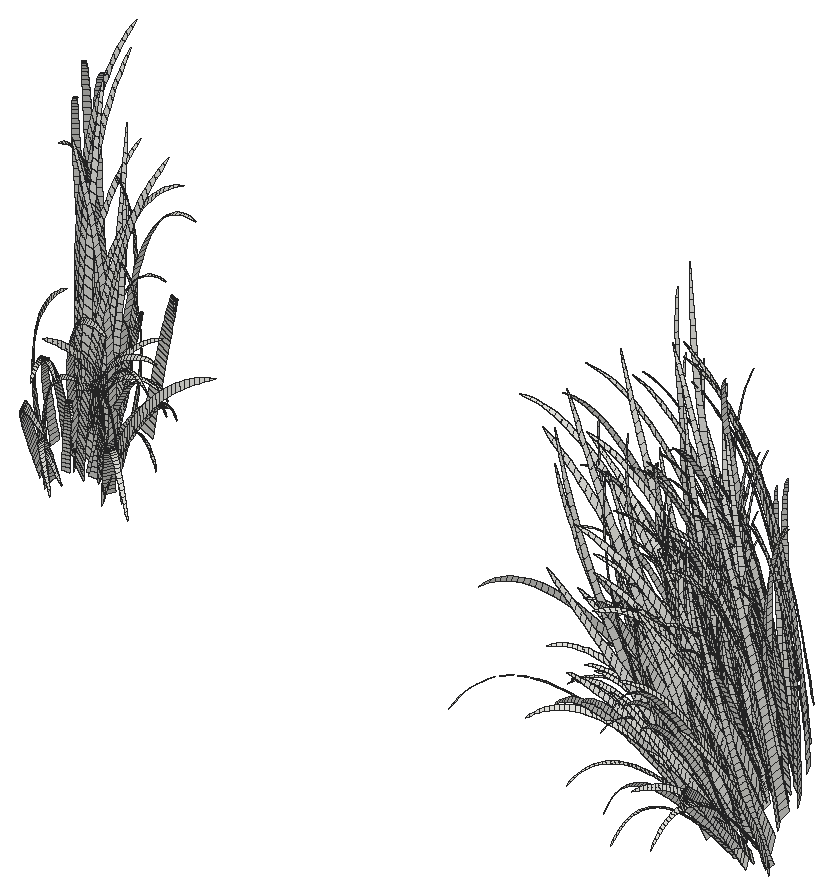
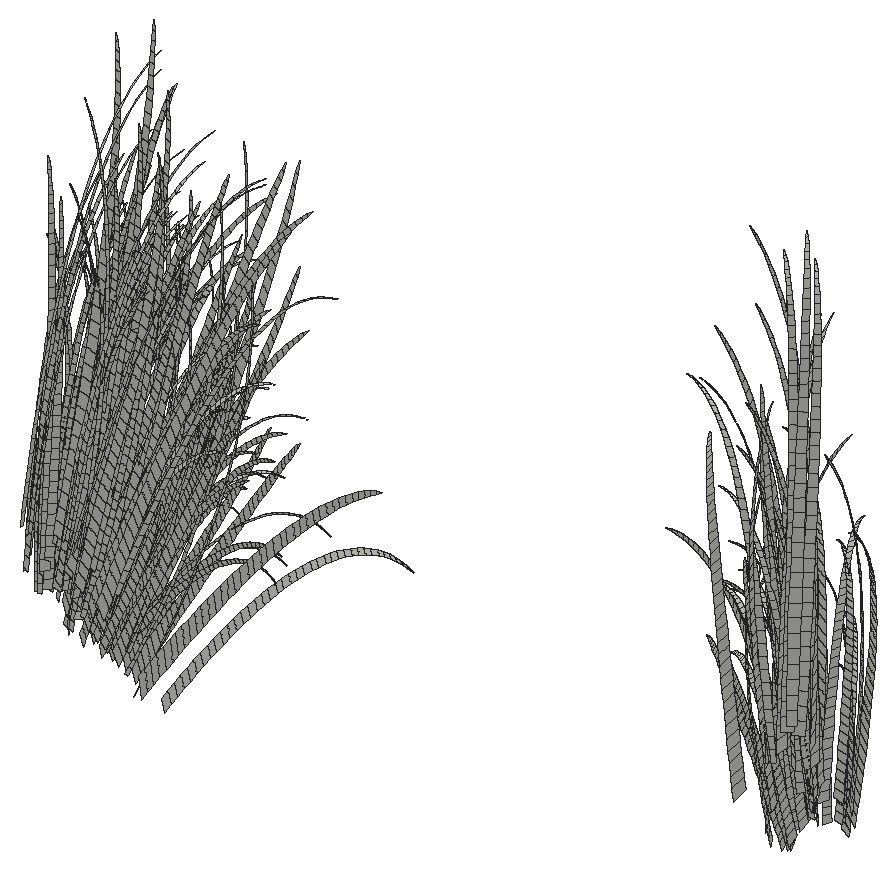
# SketchUp Ruby script. Lengths in inches.
U = 1.inch
M = Sketchup.active_model
def pt(a) = Geom::Point3d.new(a.map { |v| v * U })
def face(e, loops, mat)
  f = e.add_face(loops[0].map { |a| pt(a) })
  loops[1..].each { |l| e.add_face(l.map { |a| pt(a) }).erase! }
  f.material = f.back_material = mat if mat
  f
end
# faces: each face lists its corners as indices into pts; further lists are holes
def faces(e, pts, list, mat = nil) = list.each { |f| face(e, (f[0].is_a?(Array) ? f : [f]).map { |l| l.map { |i| pts[i] } }, mat) }
# xy, xz, yz: faces in a plane at the given z, y or x. An outline is a flat list of corners, or four numbers for a rectangle; further outlines are holes
def ring(l) = l.size == 4 ? [[l[0], l[1]], [l[2], l[1]], [l[2], l[3]], [l[0], l[3]]] : l.each_slice(2).to_a
def flat(e, list, mat, &to3) = list.each { |f| face(e, (f[0].is_a?(Array) ? f : [f]).map { |l| ring(l).map { |u, v| to3.(u, v) } }, mat) }
def xy(e, z, list, mat = nil) = flat(e, list, mat) { |x, y| [x, y, z] }
def xz(e, y, list, mat = nil) = flat(e, list, mat) { |x, z| [x, y, z] }
def yz(e, x, list, mat = nil) = flat(e, list, mat) { |y, z| [x, y, z] }
def lines(e, pts, list) = list.each { |a, b| e.add_line(pt(pts[a]), pt(pts[b])) }
# prism: a flat outline (further loops are holes) pulled along v
def prism(e, loops, v, mat = nil)
  f = face(e, loops, mat); d = Geom::Vector3d.new(v.map { |x| x * U })
  f.pushpull(f.normal.samedirection?(d) ? d.length : -d.length)
end
def box(e, o, s, mat = nil) = prism(e, [[o, [o[0] + s[0], o[1], o[2]], [o[0] + s[0], o[1] + s[1], o[2]], [o[0], o[1] + s[1], o[2]]]], [0, 0, s[2]], mat)
def at(x, y, z, deg = 0) = Geom::Transformation.translation(pt([x, y, z])) * Geom::Transformation.rotation(ORIGIN, Z_AXIS, deg.degrees)
def axes(o, x, y, z) = Geom::Transformation.new([*x, 0, *y, 0, *z, 0, *pt(o).to_a, 1])
def part(name) = M.definitions.add(name)
# library, detail: a bought-in or finely detailed component or shape, given as its bounding box
def library(name, o, s) = part(name).tap { |d| box(d.entities, o, s) }
def detail(e, o, s) = box(e.add_group.entities, o, s)
def put(e, d, t, mat = nil) = e.add_instance(d, t).tap { |i| i.material = mat if mat }
def group(e, t, mat = nil) = e.add_group.tap { |g| g.transformation = t; g.material = mat if mat }.entities
root = M.entities
c1 = part("fur_instance\#8")
p = [[-0.25,1.49,0.03],[0.25,-1.49,-0.03],[0.44,-1.47,1.51],[-0.05,1.47,1.57],[0.65,-1.44,3.05],[0.16,1.45,3.11],
  [0.86,-1.42,4.59],[0.38,1.44,4.65],[1.1,-1.39,6.13],[0.62,1.43,6.18],[1.34,-1.35,7.66],[0.875,1.42,7.72],
  [1.6,-1.32,9.19],[1.14,1.41,9.25],[1.88,-1.28,10.72],[1.43,1.41,10.78],[2.18,-1.24,12.25],[1.73,1.41,12.3],
  [2.49,-1.19,13.77],[2.05,1.41,13.82],[2.83,-1.15,15.29],[2.4,1.41,15.34],[3.18,-1.09,16.8],[2.76,1.42,16.85],
  [3.56,-1.03,18.31],[3.14,1.43,18.35],[3.96,-0.97,19.81],[3.55,1.44,19.85],[4.38,-0.91,21.3],[3.99,1.46,21.35],
  [4.84,-0.83,22.78],[4.45,1.48,22.83],[5.32,-0.76,24.26],[4.93,1.51,24.31],[5.82,-0.67,25.73],[5.45,1.54,25.77],
  [6.36,-0.59,27.18],[6,1.57,27.23],[6.93,-0.49,28.625],[6.58,1.61,28.67],[7.54,-0.39,30.05],[7.19,1.66,30.1],
  [8.18,-0.28,31.47],[7.84,1.71,31.51],[8.85,-0.16,32.86],[8.53,1.77,32.9],[9.57,-0.04,34.24],[9.25,1.83,34.27],
  [10.32,0.09,35.59],[10.02,1.9,35.625],[11.12,0.23,36.92],[10.82,1.97,36.95],[11.95,0.38,38.22],[11.67,2.06,38.25],
  [12.84,0.54,39.49],[12.57,2.14,39.52],[13.76,0.71,40.73],[13.51,2.24,40.76],[14.73,0.89,41.93],[14.49,2.34,41.95],
  [15.75,1.08,43.09],[15.52,2.45,43.11],[16.82,1.28,44.2],[16.6,2.5625,44.23],[17.93,1.5,45.27],[17.73,2.68,45.29],
  [19.08,1.73,46.28],[18.9,2.81,46.3],[20.29,1.97,47.24],[20.125,2.93,47.26],[21.53,2.22,48.13],[21.39,3.0625,48.15],
  [22.82,2.5,48.96],[22.7,3.1875,48.98],[24.14,2.8125,49.72],[24.06,3.3,49.73],[25.48,3.27,50.41]]
faces(c1.entities,p,[[0,1,2,3],[3,2,4,5],[5,4,6,7],[7,6,8,9],[9,8,10,11],[11,10,12,13],[13,12,14,15],[15,14,16,17],
  [17,16,18,19],[19,18,20,21],[21,20,22,23],[23,22,24,25],[25,24,26,27],[27,26,28,29],[29,28,30,31],[31,30,32,33],
  [33,32,34,35],[35,34,36,37],[37,36,38,39],[39,38,40,41],[41,40,42,43],[43,42,44,45],[45,44,46,47],[47,46,48,49],
  [49,48,50,51],[51,50,52,53],[53,52,54,55],[55,54,56,57],[57,56,58,59],[59,58,60,61],[61,60,62,63],[63,62,64,65],
  [65,64,66,67],[67,66,68,69],[69,68,70,71],[71,70,72,73],[73,72,74,75],[75,74,76]])
put(root,c1,axes([50.95,63.79,4.28],[0.19476,0.01919,-0.07142],[-0.00771,0.11743,0.2824],[0.0412,-0.14851,0.33769]))
put(root,c1,axes([51.41,68.37,11.2],[0.12423,-0.19532,-0.16493],[0.21975,0.1108,-0.06089],[0.05484,-0.10226,0.55089]))
put(root,c1,axes([51.72,65.86,7.6],[0.10368,0.16194,0.09463],[-0.18699,0.06759,0.22582],[0.06767,-0.12287,0.43828]))
put(root,c1,axes([51.52,63.51,2.55],[0.10797,-0.02278,-0.25368],[0.09924,0.08349,0.12145],[0.06318,-0.1256,0.22064]))
put(root,c1,axes([51.4,64.28,4.91],[0.12346,-0.06874,-0.2664],[0.133,0.10274,0.08323],[0.06093,-0.13474,0.32518]))
put(root,c1,axes([52.49,67.7,9.01],[-0.03736,-0.20284,-0.08426],[0.21276,-0.01244,-0.24024],[0.09664,-0.09898,0.46456]))
put(root,c1,axes([51.6,67.38,10.11],[0.143,-0.17445,-0.17187],[0.20045,0.12222,-0.01071],[0.04373,-0.10813,0.53269]))
put(root,c1,axes([51.36,63.54,3.02],[0.15494,0.00054,-0.15254],[0.03594,0.10834,0.19122],[0.0534,-0.11809,0.285]))
put(root,c1,axes([51.67,65.4,6.25],[0.10826,0.14171,0.01778],[-0.14869,0.07846,0.21324],[0.07154,-0.09642,0.38649]))
put(root,c1,axes([52.34,64.39,4.52],[0.01148,-0.14011,-0.26001],[0.19146,0.05137,-0.16224],[0.08794,-0.13547,0.35942]))
put(root,c1,axes([52.12,64.33,3.29],[0.05454,-0.09644,-0.21571],[0.13016,0.08062,-0.0942],[0.08114,-0.09154,0.27821]))
put(root,c1,axes([51.49,68.5,10.89],[0.15717,-0.16888,-0.16909],[0.19008,0.14007,-0.03029],[0.05359,-0.09991,0.53827]))
put(root,c1,axes([53.4,65.53,4.23],[-0.06239,0.13265,0.23168],[-0.15342,-0.10065,0.1704],[0.112,-0.09352,0.34293]))
put(root,c1,axes([53.05,67.65,5.39],[-0.06465,-0.16754,0.157],[0.14103,-0.07728,-0.22676],[0.11827,-0.02606,0.33858]))
put(root,c1,axes([51.23,63.45,3.46],[0.19478,-0.02841,-0.30734],[0.1247,0.10642,0.29017],[0.06226,-0.20052,0.32988]))
put(root,c1,axes([51.875,63.57,3.06],[0.10305,-0.05896,-0.3685],[0.16571,0.09891,0.06527],[0.08407,-0.16713,0.29358]))
put(root,c1,axes([51.74,66.04,8.76],[0.19083,0.13184,0.05677],[-0.15811,0.13743,0.27367],[0.05817,-0.15117,0.49659]))
put(root,c1,axes([52.2,65.21,5.21],[0.13121,0.11551,-0.02739],[-0.11587,0.10209,0.2018],[0.06808,-0.09176,0.36783]))
put(root,c1,axes([52.48,66.79,3.14],[0.04832,-0.14518,0.00787],[0.12065,0.04323,-0.22286],[0.09094,-0.00311,0.27632]))
put(root,c1,axes([53.33,64.8125,4.59],[-0.00332,0.15612,0.27725],[-0.2105,-0.04955,0.19049],[0.09652,-0.14869,0.3945]))
put(root,c1,axes([52.45,65.87,3.61],[0.0496,-0.12974,-0.10453],[0.11629,0.07093,-0.20268],[0.09864,-0.03996,0.27723]))
put(root,c1,axes([53,66.11,2.42],[-0.03175,-0.14429,0.13902],[0.10175,-0.04851,-0.23869],[0.11949,-0.01479,0.22844]))
put(root,c1,axes([53.34,65.14,3.1875],[-0.05491,0.09737,0.28251],[-0.12379,-0.11722,0.16383],[0.12913,-0.0934,0.26231]))
put(root,c1,axes([53.54,65.13,3.01],[-0.0662,0.08995,0.30205],[-0.12202,-0.12772,0.14438],[0.13238,-0.09575,0.2689]))
put(root,c1,axes([54.47,65.6,4],[-0.14869,0.01051,0.38769],[-0.10168,-0.16677,-0.09879],[0.14048,-0.14032,0.31849]))
put(root,c1,axes([52.32,64.83,3.52],[0.12216,0.08749,-0.1288],[-0.05725,0.10364,0.19567],[0.09123,-0.07618,0.27934]))
put(root,c1,axes([53.6,65.27,3.09],[-0.06626,-0.1567,-0.04431],[0.12258,-0.00555,-0.33309],[0.13287,-0.09611,0.2699]))
put(root,c1,axes([53.87,66.85,2.61],[-0.09134,-0.12785,0.22656],[0.07697,-0.11104,-0.22116],[0.1384,-0.04262,0.25929]))
put(root,c1,axes([53.06,64.43,3.43],[0.07572,0.13089,0.20219],[-0.15985,-0.01369,0.30106],[0.10643,-0.14683,0.2864]))
put(root,c1,axes([52.45,66.13,5.8],[0.16409,-0.04331,-0.20606],[0.05728,0.16704,-0.00737],[0.08461,-0.06565,0.38043]))
put(root,c1,axes([52.86,66.375,2.64],[0.06266,-0.1249,-0.10853],[0.0861,0.08678,-0.25374],[0.11938,-0.01478,0.22823]))
put(root,c1,axes([52.64,64.99,3.71],[0.14109,0.00407,-0.23949],[0.03377,0.14579,0.07817],[0.0981,-0.08192,0.30039]))
put(root,c1,axes([52.9,65.55,4.3],[0.12005,-0.06141,-0.26447],[0.09556,0.14151,-0.0324],[0.10376,-0.08664,0.31771]))
put(root,c1,axes([52.77,64.79,3.9375],[0.16454,0.02683,-0.22071],[0.01929,0.1451,0.16624],[0.09525,-0.10745,0.32659]))
put(root,c1,axes([55.3,65.3,2.58],[-0.15559,-0.16713,0.03304],[0.11706,-0.06849,-0.43118],[0.15185,-0.15167,0.34426]))
put(root,c1,axes([53.23,66.41,2.55],[0.068,-0.12804,-0.12081],[0.08818,0.09434,-0.26208],[0.12484,-0.01545,0.23865]))
put(root,c1,axes([52.68,66.45,7.34],[0.20769,0.04966,-0.15926],[-0.03101,0.17814,0.18526],[0.08167,-0.11008,0.44127]))
put(root,c1,axes([53.27,65.6,2.96],[0.06859,-0.09014,-0.25373],[0.09618,0.12505,-0.16822],[0.12923,-0.06487,0.24688]))
put(root,c1,axes([52.79,64.54,5.12],[0.20792,-0.04098,-0.29203],[0.11115,0.15527,0.21492],[0.07916,-0.17504,0.42246]))
put(root,c1,axes([53.32,65.61,3.51],[0.12063,-0.06515,-0.25144],[0.08341,0.14829,-0.07405],[0.10987,-0.06634,0.31554]))
put(root,c1,axes([53.49,65.05,5.17],[0.15805,0.15051,0.05502],[-0.15454,0.08321,0.34889],[0.10135,-0.15612,0.41421]))
put(root,c1,axes([53.62,67.2,7.69],[0.20327,-0.05604,-0.25675],[0.08292,0.19878,0.03195],[0.09822,-0.10059,0.47212]))
put(root,c1,axes([54.89,64.87,2.58],[0.10396,-0.07911,-0.43973],[0.18772,0.13868,-0.01375],[0.12911,-0.17813,0.34745]))
put(root,c1,axes([55.28,67.78,5.36],[0.04979,-0.1895,-0.18773],[0.18438,0.09265,-0.2851],[0.14308,-0.0864,0.41092]))
put(root,c1,axes([54.38,64.82,2.28],[0.1674,0.12348,-0.15342],[-0.05527,0.10723,0.36025],[0.13749,-0.13733,0.3117]))
put(root,c1,axes([95.04,68.76,-1.625],[-0.02161,-0.16628,-0.28389],[0.16425,-0.14433,0.32408],[-0.18224,-0.08282,0.344]))
put(root,c1,axes([95.1,66.78,-3.61],[-0.07933,-0.07892,-0.44402],[0.19255,-0.17562,0.06989],[-0.14788,-0.14983,0.35337]))
put(root,c1,axes([97.78,67.33,2.39],[-0.23554,0.05296,-0.19778],[0.0198,-0.2043,-0.19606],[-0.09324,-0.11985,0.49597]))
put(root,c1,axes([97.57,68.95,2.17],[-0.04128,-0.19919,-0.10991],[0.2038,-0.09544,0.23105],[-0.11682,-0.05581,0.46862]))
put(root,c1,axes([96.75,67.08,-3.375],[0.13283,-0.0342,0.36955],[-0.05695,0.18902,0.06859],[-0.15898,-0.07225,0.3001]))
put(root,c1,axes([99.71,64.83,-2.87],[-0.12873,0.10197,-0.18861],[-0.01018,-0.10343,-0.24101],[-0.11719,-0.08155,0.24232]))
put(root,c1,axes([98.99,68.05,1.3],[-0.08516,-0.14739,-0.15062],[0.16457,-0.13044,0.17116],[-0.1041,-0.04973,0.41758]))
put(root,c1,axes([99.8,64.22,-2.46],[-0.15935,0.03269,-0.28558],[0.09029,-0.13292,-0.22683],[-0.09601,-0.14239,0.28508]))
put(root,c1,axes([99.8,64.65,-3.17],[-0.14081,0.09765,-0.1356],[-0.01218,-0.08683,-0.27326],[-0.10036,-0.10168,0.23982]))
put(root,c1,axes([99.95,66.09,1.125],[-0.18347,0.1171,-0.07334],[-0.07461,-0.13251,-0.22152],[-0.07812,-0.10043,0.41558]))
put(root,c1,axes([99.83,64.51,-2.67],[-0.15082,0.11254,-0.07354],[-0.05779,-0.09193,-0.25822],[-0.08893,-0.09949,0.31347]))
put(root,c1,axes([99.8125,66.52,0.57],[-0.149,-0.04647,-0.21352],[0.09287,-0.17245,0.02054],[-0.09229,-0.06322,0.38876]))
put(root,c1,axes([99.33,64.27,-2.34],[-0.09966,0.12678,0.30336],[-0.19172,0.0268,-0.26785],[-0.07616,-0.17634,0.31506]))
put(root,c1,axes([98.57,66.42,-2.16],[0.05365,-0.16969,-0.03778],[0.13986,-0.00916,0.27148],[-0.1167,-0.06341,0.32492]))
put(root,c1,axes([100.03,64.77,-2.5],[-0.10552,0.13111,0.03774],[-0.1075,-0.03434,-0.24755],[-0.08294,-0.09279,0.29236]))
put(root,c1,axes([100.58,64.85,1.03],[-0.23362,0.09843,0.07428],[-0.08627,-0.11761,-0.36241],[-0.04076,-0.18596,0.42692]))
put(root,c1,axes([99.77,65.09,-2.79],[-0.05906,0.14196,0.06951],[-0.12604,0.00717,-0.23329],[-0.09379,-0.07416,0.28621]))
put(root,c1,axes([98.48,65.05,-3.62],[0.08197,-0.14846,-0.17255],[0.1435,-0.03613,0.3122],[-0.11735,-0.1189,0.28043]))
put(root,c1,axes([100.61,67.41,4.04],[-0.2227,-0.02851,-0.13015],[0.07795,-0.20389,-0.10631],[-0.04666,-0.10194,0.51151]))
put(root,c1,axes([100,65.87,-2.4375],[-0.05395,-0.10392,-0.15053],[0.10796,-0.10426,0.17042],[-0.10255,-0.03484,0.272]))
put(root,c1,axes([100.59,64.13,-1.74],[-0.17727,0.00029,-0.20455],[0.08516,-0.1353,-0.21935],[-0.05731,-0.14134,0.34686]))
put(root,c1,axes([100.34,64.61,-1.87],[-0.10062,-0.049,-0.26041],[0.12035,-0.13237,-0.01381],[-0.08638,-0.09663,0.30447]))
put(root,c1,axes([100.65,66.22,-1.26],[-0.12457,-0.03797,-0.15408],[0.05979,-0.14532,0.07008],[-0.07901,-0.02356,0.31353]))
put(root,c1,axes([100.29,64.01,-1.29],[-0.15374,0.14658,0.25603],[-0.19784,-0.04817,-0.27014],[-0.04101,-0.18709,0.42951]))
put(root,c1,axes([98.68,65.41,-3.61],[0.13307,-0.06357,0.27984],[-0.03809,0.14212,0.17121],[-0.12562,-0.08741,0.25976]))
put(root,c1,axes([100.56,64.3,-3],[-0.0986,0.1202,0.03133],[-0.09749,-0.03341,-0.22837],[-0.07635,-0.08541,0.26912]))
put(root,c1,axes([100.35,64.0625,-3.4],[-0.08725,-0.02366,-0.29756],[0.12591,-0.11202,-0.06714],[-0.0803,-0.1191,0.23844]))
put(root,c1,axes([100.88,64.14,-2.43],[-0.15103,0.03829,-0.1475],[0.02836,-0.11444,-0.19385],[-0.06472,-0.10394,0.28282]))
put(root,c1,axes([98.18,65.9,-1.8125],[0.17403,-0.06722,0.24815],[-0.01797,0.16553,0.179],[-0.11789,-0.09322,0.35975]))
put(root,c1,axes([99.85,63.5625,-3.42],[-0.07738,0.12181,0.42116],[-0.24475,0.02807,-0.19007],[-0.04925,-0.2161,0.35893]))
put(root,c1,axes([101.0625,63.58,-2.42],[-0.19758,0.0885,0.1271],[-0.09447,-0.05952,-0.37318],[-0.04202,-0.18438,0.30623]))
put(root,c1,axes([99.55,65.45,-1.95],[0.04667,0.10587,0.22641],[-0.14224,0.11026,-0.13144],[-0.10087,-0.07976,0.30781]))
put(root,c1,axes([100.4375,65,0.8],[-0.12023,0.16893,0.15811],[-0.19192,-0.04724,-0.20175],[-0.05017,-0.13536,0.45159]))
put(root,c1,axes([100.7,64.82,-0.86],[-0.1513,-0.02821,-0.17374],[0.08683,-0.1419,-0.10144],[-0.05423,-0.09755,0.35603]))
put(root,c1,axes([100.82,64.62,-1.9375],[-0.07947,0.12548,0.07397],[-0.11521,-0.01055,-0.22059],[-0.07706,-0.08621,0.27164]))
put(root,c1,axes([100.52,66.85,-1.51],[-0.06439,-0.12354,-0.04587],[0.12333,-0.08786,0.16125],[-0.07712,-0.0102,0.31415]))
put(root,c1,axes([99.97,65.11,-2.89],[0.02731,-0.14018,-0.06519],[0.12315,-0.02871,0.2214],[-0.09827,-0.0534,0.27359]))
put(root,c1,axes([99.37,64.66,-3.49],[0.09631,-0.13966,-0.10726],[0.11682,-0.00954,0.30869],[-0.10751,-0.10893,0.25692]))
put(root,c1,axes([101.3,64.74,-0.29],[-0.18173,0.02045,-0.09763],[0.0261,-0.14072,-0.18343],[-0.04068,-0.10974,0.36609]))
put(root,c1,axes([99.78,65.89,-2.1],[0.06905,-0.15041,0.07394],[0.1069,0.0384,0.22809],[-0.10814,-0.03674,0.28683]))
put(root,c1,axes([99.75,66.28,-0.53],[0.02994,-0.16585,-0.05499],[0.16129,-0.01842,0.19273],[-0.08623,-0.05907,0.36324]))
put(root,c1,axes([101.38,63.5,-2.85],[-0.18497,0.04944,-0.02341],[-0.00878,-0.07542,-0.33252],[-0.03553,-0.1559,0.25894]))
put(root,c1,axes([101.1,65.75,0.07],[-0.14413,-0.05167,-0.11933],[0.08701,-0.14734,-0.01287],[-0.04763,-0.0596,0.37283]))
put(root,c1,axes([100.82,63.85,-3.23],[-0.04193,0.09854,0.23039],[-0.14173,0.04993,-0.18317],[-0.07748,-0.11492,0.23007]))
put(root,c1,axes([100.58,66.04,-1.19],[-0.02354,-0.13666,-0.06934],[0.13862,-0.06024,0.1585],[-0.07899,-0.03774,0.31687]))
put(root,c1,axes([101.54,63.625,-2.79],[-0.15528,0.03655,-0.09389],[0.01601,-0.10098,-0.21878],[-0.04549,-0.11219,0.27533]))
put(root,c1,axes([101.57,64.46,-1.24],[-0.15238,0.03287,-0.097],[0.00948,-0.12228,-0.14695],[-0.04746,-0.08538,0.3116]))
put(root,c1,axes([100.82,65.7,-0.79],[-0.02967,-0.13006,-0.11002],[0.14258,-0.07093,0.13984],[-0.07655,-0.05244,0.32247]))
put(root,c1,axes([99.69,65.01,-2.43],[0.10962,-0.14134,0.02858],[0.09848,0.05163,0.25611],[-0.09929,-0.07851,0.30299]))
put(root,c1,axes([101.19,65.02,-0.08],[-0.07622,0.14548,0.11566],[-0.15943,-0.01772,-0.1678],[-0.05494,-0.09882,0.36066]))
put(root,c1,axes([101.91,65.69,2.6875],[-0.23536,0.00031,-0.04255],[0.03502,-0.16941,-0.26023],[-0.00865,-0.15175,0.46324]))
put(root,c1,axes([100.29,63.92,-3.33],[0.07176,0.04443,0.32956],[-0.1495,0.11571,0.02095],[-0.08693,-0.12893,0.25813]))
put(root,c1,axes([101.4375,67.92,3.42],[-0.16552,-0.11118,-0.05649],[0.14207,-0.16762,-0.00154],[-0.02412,-0.05905,0.48802]))
put(root,c1,axes([101.4,63.68,-1.98],[-0.1192,0.12425,0.22535],[-0.17166,-0.03356,-0.21354],[-0.0342,-0.15606,0.35826]))
put(root,c1,axes([101.11,65.45,-0.76],[-0.02927,-0.12714,-0.10789],[0.13946,-0.06963,0.13664],[-0.0749,-0.05131,0.31553]))
put(root,c1,axes([99.36,64.84,-1.2],[0.13498,-0.15634,-0.12045],[0.15269,0.03421,0.29976],[-0.08583,-0.13785,0.37509]))
put(root,c1,axes([100.6,66.07,2.55],[-0.00008,0.17023,0.2439],[-0.22913,0.05018,-0.08813],[-0.05076,-0.13695,0.4569]))
put(root,c1,axes([99.43,66.21,0.12],[0.15632,-0.13539,0.07566],[0.09629,0.11232,0.20743],[-0.0859,-0.08088,0.3964]))
put(root,c1,axes([99.32,63.875,-3.22],[0.17581,0.00429,0.35889],[-0.15371,0.13999,0.25001],[-0.08231,-0.1906,0.34052]))
put(root,c1,axes([100.51,65.44,0.9],[0.05112,0.14176,0.22694],[-0.19757,0.09246,-0.06236],[-0.06344,-0.11412,0.4165]))
put(root,c1,axes([100.85,65.46,-0.4],[0.0229,-0.1484,-0.09458],[0.15576,-0.02704,0.16403],[-0.07366,-0.06935,0.33993]))
put(root,c1,axes([101.13,67.02,2.6],[-0.04613,-0.168,-0.12838],[0.20048,-0.07761,0.07112],[-0.05022,-0.08162,0.45074]))
put(root,c1,axes([100.65,66.9375,1.67],[0.01336,-0.18156,-0.05149],[0.1916,-0.02315,0.12623],[-0.05991,-0.05859,0.42926]))
put(root,c1,axes([100.2,65.12,-2.0625],[0.13306,-0.03251,0.2141],[-0.03468,0.1366,0.1095],[-0.09265,-0.07326,0.28274]))
put(root,c1,axes([101.7,65.3,1.17],[-0.14651,-0.09517,-0.11625],[0.13838,-0.13795,-0.08263],[-0.01824,-0.0963,0.42995]))
put(root,c1,axes([102.42,66.82,3.63],[-0.22374,-0.02944,-0.01516],[0.05551,-0.18692,-0.16154],[0.00543,-0.11272,0.49003]))
put(root,c1,axes([101.31,63.75,-2.29],[-0.00857,-0.10681,-0.26092],[0.17656,-0.05814,0.06779],[-0.05152,-0.12704,0.31177]))
put(root,c1,axes([100.22,64.66,-1.64],[0.14194,0.01295,0.23971],[-0.09799,0.13483,0.13149],[-0.07264,-0.11667,0.31745]))
put(root,c1,axes([101.08,64.1875,-2.09],[0.04246,-0.11664,-0.17724],[0.14637,-0.02684,0.16417],[-0.06419,-0.10309,0.2805]))
put(root,c1,axes([102.23,66.82,1.88],[-0.13872,-0.10688,-0.05008],[0.13478,-0.14007,-0.01499],[-0.01621,-0.05768,0.43132]))
put(root,c1,axes([101.87,67.18,1.63],[-0.09202,-0.14419,-0.02135],[0.16494,-0.10399,0.03603],[-0.02333,-0.03794,0.42396]))
put(root,c1,axes([101.05,66.01,-0.76],[0.09225,-0.12894,0.11038],[0.10291,0.0771,0.12838],[-0.07903,-0.02356,0.31361]))
put(root,c1,axes([101.19,63.42,-3.625],[0.04168,-0.09258,-0.28201],[0.16554,-0.04371,0.15063],[-0.06017,-0.13932,0.24891]))
put(root,c1,axes([100.35,64.72,-1.42],[0.15549,-0.01208,0.20833],[-0.06905,0.13306,0.17126],[-0.07165,-0.11508,0.31313]))
put(root,c1,axes([102.73,65.93,1.71],[-0.18618,-0.03996,-0.02577],[0.06509,-0.15689,-0.1364],[0.00464,-0.09644,0.41925]))
put(root,c1,axes([102.74,65.55,0.29],[-0.15853,0.06077,0.01255],[-0.05151,-0.13731,-0.04414],[-0.00488,-0.05314,0.37046]))
put(root,c1,axes([103.16,64.09,-0.1],[-0.25079,-0.01126,0.01167],[0.02691,-0.14432,-0.37072],[0.02191,-0.19373,0.42855]))
put(root,c1,axes([102.62,63.75,-1.61],[-0.15193,-0.01941,-0.09588],[0.0644,-0.09304,-0.22233],[-0.00624,-0.12588,0.27933]))
put(root,c1,axes([102.92,62.98,-3.875],[-0.16406,0.03446,0.0684],[-0.03839,-0.06194,-0.29017],[-0.00638,-0.14462,0.2315]))
put(root,c1,axes([100.02,63.98,-3.04],[0.18766,-0.05407,0.15304],[-0.0375,0.10124,0.3241],[-0.06745,-0.15619,0.27904]))
put(root,c1,axes([101.72,65.78,3.08],[-0.04308,0.17847,0.273],[-0.24701,-0.00413,-0.05166],[-0.00912,-0.15991,0.48813]))
put(root,c1,axes([101.09,64.11,-1.17],[0.03417,-0.12525,-0.29157],[0.20378,-0.0224,0.09589],[-0.03382,-0.15429,0.3542]))
put(root,c1,axes([101.375,64.54,0.17],[0.00591,-0.15376,-0.2335],[0.21361,-0.03099,0.04882],[-0.02765,-0.13326,0.41924]))
put(root,c1,axes([102.18,64.44,0.12],[-0.06192,0.14505,0.21697],[-0.19671,-0.02273,-0.07174],[-0.0075,-0.13152,0.40147]))
put(root,c1,axes([103.42,63.75,-1.2],[-0.22603,-0.01056,0.00948],[0.02497,-0.13008,-0.33426],[0.01976,-0.17466,0.38636]))
put(root,c1,axes([101.9375,65.36,1.6],[0.0038,0.14954,0.23139],[-0.20994,0.03733,-0.03743],[-0.02717,-0.13094,0.41195]))
put(root,c1,axes([102.04,65.625,-0.19],[-0.04654,-0.13259,-0.03011],[0.14978,-0.05997,0.02545],[-0.01873,-0.03986,0.3514]))
put(root,c1,axes([102.08,63.08,-3.89],[-0.02123,-0.06781,-0.31584],[0.17417,-0.05199,-0.00113],[-0.03366,-0.14772,0.24534]))
put(root,c1,axes([102.95,64.51,0.86],[-0.18897,-0.07724,-0.16578],[0.14014,-0.11074,-0.30364],[0.02044,-0.18069,0.39971]))
put(root,c1,axes([102.11,65.26,1.11],[-0.0211,0.16438,0.13367],[-0.19675,0.00758,-0.04177],[-0.01791,-0.09455,0.42215]))
put(root,c1,axes([102.77,66.02,1.41],[-0.1296,-0.11177,-0.03307],[0.13714,-0.12794,-0.0397],[-0.00189,-0.06022,0.41924]))
put(root,c1,axes([101.6,63.68,-2.53],[0.0606,-0.10906,-0.18612],[0.14677,-0.00638,0.15494],[-0.04628,-0.11412,0.28007]))
put(root,c1,axes([103.19,65.31,2.02],[-0.15736,0.12863,0.21317],[-0.17096,-0.10355,-0.14422],[0.01307,-0.14881,0.45294]))
put(root,c1,axes([103.13,64.49,-0.17],[-0.16225,-0.04777,-0.05886],[0.07812,-0.11873,-0.19059],[0.01013,-0.11533,0.35104]))
put(root,c1,axes([102.96,65.42,0.84],[-0.13495,-0.09194,-0.07228],[0.12419,-0.11921,-0.10694],[0.00432,-0.08968,0.38985]))
put(root,c1,axes([102.11,66.05,1.61],[-0.00432,-0.15952,-0.128],[0.19173,-0.03266,0.04648],[-0.02798,-0.08806,0.41192]))
put(root,c1,axes([101.64,63.94,-1.72],[0.10535,0.0488,0.23666],[-0.12967,0.10407,0.09442],[-0.04869,-0.12008,0.29468]))
put(root,c1,axes([102.11,66.96,1.06],[-0.00822,-0.16722,0.01164],[0.17876,-0.02595,0.03382],[-0.01925,-0.0303,0.40131]))
put(root,c1,axes([103.25,64.4,-0.72],[-0.14242,0.06423,0.07833],[-0.06984,-0.11466,-0.07925],[0.01251,-0.07634,0.33832]))
put(root,c1,axes([103.3,64.98,0.65],[-0.1422,0.11091,0.11586],[-0.12628,-0.11191,-0.06649],[0.015,-0.09153,0.40561]))
put(root,c1,axes([103.55,67.46,2.98],[-0.17633,-0.09809,0.01724],[0.1199,-0.16919,-0.04915],[0.01352,-0.05835,0.47546]))
put(root,c1,axes([103.33,63.61,-1.84],[-0.13701,0.06738,0.19305],[-0.11347,-0.07671,-0.17654],[0.01546,-0.13663,0.30225]))
put(root,c1,axes([103.31,65.19,0.11],[-0.14765,0.06695,0.09599],[-0.07527,-0.12279,-0.06548],[0.02169,-0.07701,0.35566]))
put(root,c1,axes([103.68,67.52,4.05],[-0.22223,-0.05187,0.06437],[0.06185,-0.19269,-0.14793],[0.04097,-0.1013,0.49904]))
put(root,c1,axes([101.3125,66.37,0.56],[0.1666,-0.05285,0.10887],[0.0248,0.15525,0.04679],[-0.05548,-0.04238,0.37888]))
put(root,c1,axes([103.2,63.07,-3.46],[-0.13424,-0.03889,-0.12787],[0.08866,-0.05443,-0.25596],[0.01839,-0.13945,0.22254]))
put(root,c1,axes([102.41,64.55,-0.3],[0.0286,0.11518,0.18982],[-0.16763,0.04809,-0.0018],[-0.022,-0.10604,0.33361]))
put(root,c1,axes([101.83,64.7,-0.68],[0.09089,0.09523,0.11248],[-0.12952,0.09997,0.00707],[-0.03129,-0.06837,0.34303]))
put(root,c1,axes([102.57,64.97,-0.26],[0.0055,0.12915,0.11043],[-0.15799,0.02454,-0.01796],[-0.01431,-0.07554,0.33727]))
put(root,c1,axes([100.84,66.85,2.46],[0.2061,-0.01344,0.1131],[-0.02793,0.18662,0.09605],[-0.05077,-0.08252,0.4557]))
put(root,c1,axes([102.77,63.37,-2.53],[-0.02267,0.09523,0.24051],[-0.16406,0.00552,-0.03477],[-0.00627,-0.12634,0.28034]))
put(root,c1,axes([101.66,65.7,0.39],[0.13539,0.06511,0.11886],[-0.10233,0.13809,0.02305],[-0.04143,-0.06734,0.37184]))
put(root,c1,axes([103.5,66.6,1.33],[-0.12883,-0.11449,0.01319],[0.1336,-0.12723,-0.04151],[0.01291,-0.04776,0.41418]))
put(root,c1,axes([101.93,66.85,4.24],[0.02992,-0.20268,-0.17218],[0.24479,0.00013,0.02509],[-0.00825,-0.12029,0.52424]))
put(root,c1,axes([103.52,67.86,2.1875],[-0.11995,-0.14094,0.03187],[0.15995,-0.12378,-0.02155],[0.01135,-0.03745,0.44662]))
put(root,c1,axes([103.59,68.1,4.86],[-0.1863,-0.12854,0.00057],[0.15019,-0.16226,-0.16735],[0.0425,-0.10509,0.5177]))
put(root,c1,axes([103.1,66.31,0.7],[-0.07961,-0.13689,0.01423],[0.15313,-0.0843,-0.034],[0.01219,-0.0383,0.38556]))
put(root,c1,axes([103.09,66.73,1.11],[-0.07772,-0.14595,0.01956],[0.16231,-0.0838,-0.0308],[0.01178,-0.03674,0.40206]))
put(root,c1,axes([103.15,66.22,0.32],[-0.07124,-0.13476,0.02236],[0.14958,-0.07747,-0.02272],[0.00941,-0.03103,0.37011]))
put(root,c1,axes([102.87,63.66,-1.74],[0.01737,0.09262,0.24572],[-0.16736,0.02852,0.02395],[-0.00637,-0.12835,0.28481]))
put(root,c1,axes([101.24,67.91,4.89],[0.18706,-0.15692,-0.05371],[0.1539,0.13296,0.16341],[-0.03534,-0.11123,0.5203]))
put(root,c1,axes([101.99,64.9375,-0.48],[0.13738,0.0414,0.0972],[-0.07592,0.13055,0.05523],[-0.03104,-0.06782,0.34028]))
put(root,c1,axes([103.38,64.96,0.68],[-0.07914,0.12591,0.21103],[-0.17333,-0.05924,-0.02394],[0.02804,-0.12033,0.37519]))
put(root,c1,axes([103.48,64.61,0.05],[-0.10701,-0.11213,-0.12442],[0.15233,-0.07687,-0.16606],[0.02739,-0.11756,0.36656]))
put(root,c1,axes([104.13,64.56,-0.58],[-0.16995,0.00239,0.1052],[-0.0155,-0.13112,-0.16118],[0.04006,-0.1041,0.34197]))
put(root,c1,axes([101.97,63.27,-2.9375],[0.11054,0.06076,0.32124],[-0.18174,0.06569,0.1961],[-0.00805,-0.18258,0.29226]))
put(root,c1,axes([102.47,66.46,2.64],[0.04164,-0.17352,-0.14577],[0.20763,0.01338,0.03275],[-0.00709,-0.10329,0.45016]))
put(root,c1,axes([102.41,63.36,-2.67],[0.07036,0.07691,0.22077],[-0.15002,0.05652,0.10186],[-0.00627,-0.1264,0.28049]))
put(root,c1,axes([101.99,65.46,0.73],[0.15043,0.06237,0.10618],[-0.10193,0.14112,0.07332],[-0.02651,-0.08344,0.39031]))
put(root,c1,axes([102.07,64.57,-0.53],[0.1599,-0.01285,0.09328],[-0.0299,0.12534,0.15874],[-0.03604,-0.09723,0.32437]))
put(root,c1,axes([104.39,63.47,-2.43],[-0.19796,-0.00213,0.19119],[-0.0584,-0.09827,-0.32515],[0.05556,-0.17894,0.29438]))
put(root,c1,axes([102.91,64.5,0.05],[-0.00485,-0.13574,-0.20923],[0.19174,-0.01245,-0.03687],[0.01079,-0.12284,0.3739]))
put(root,c1,axes([101.875,64.14,-1.08],[0.16477,0.01322,0.09468],[-0.05646,0.12716,0.16983],[-0.02254,-0.10862,0.34171]))
put(root,c1,axes([104.54,66.57,1.22],[-0.18521,-0.02955,0.11381],[0.03239,-0.17376,-0.06029],[0.05035,-0.05919,0.41626]))
put(root,c1,axes([104.28,64.2,-1.51],[-0.14955,-0.02951,0.08847],[0.01953,-0.12021,-0.14832],[0.04773,-0.08667,0.30915]))
put(root,c1,axes([102.26,63.6,-2.1],[0.16669,-0.01734,0.08094],[-0.02966,0.10281,0.23812],[-0.02771,-0.12642,0.29024]))
put(root,c1,axes([102.45,63.39,-2.41],[0.12347,0.06755,0.21237],[-0.14396,0.08585,0.17984],[-0.00718,-0.14468,0.32104]))
put(root,c1,axes([104.44,65.25,1.5],[-0.16708,-0.12567,-0.06302],[0.15179,-0.11958,-0.24667],[0.05298,-0.1377,0.45233]))
put(root,c1,axes([102.56,67.21,1],[0.10751,-0.14401,0.02773],[0.14274,0.0886,-0.01156],[-0.00773,-0.0245,0.39927]))
put(root,c1,axes([103.65,63.22,-2.94],[-0.04322,-0.08103,-0.33227],[0.19342,-0.01502,-0.11763],[0.02265,-0.17179,0.27415]))
put(root,c1,axes([103.92,66.19,-0.14],[-0.08777,-0.12311,0.07978],[0.13105,-0.09185,-0.0647],[0.04014,-0.02395,0.34954]))
put(root,c1,axes([104.45,64.67,0.36],[-0.14817,-0.12463,-0.07303],[0.15181,-0.10509,-0.22784],[0.04979,-0.1294,0.42509]))
put(root,c1,axes([102.72,64.26,-0.76],[0.12885,0.05972,0.11755],[-0.10424,0.10176,0.1411],[-0.00603,-0.1057,0.32265]))
put(root,c1,axes([104.39,63.19,-3.82],[-0.14554,-0.04613,0.08103],[0.01279,-0.07284,-0.26823],[0.06295,-0.12513,0.21981]))
put(root,c1,axes([104.64,64.25,-0.79],[-0.14966,0.06135,0.2769],[-0.12806,-0.11932,-0.12286],[0.06613,-0.14624,0.35295]))
put(root,c1,axes([104.39,63.18,-3.73],[-0.08929,0.05587,0.30832],[-0.15159,-0.06244,-0.09121],[0.04736,-0.15254,0.25094]))
put(root,c1,axes([102.56,65.71,0.29],[0.16373,-0.03857,0.00921],[0.02397,0.14494,0.04432],[-0.01107,-0.05099,0.36849]))
put(root,c1,axes([103.82,65.56,0.01],[-0.04201,-0.14205,-0.02716],[0.15521,-0.03808,-0.10788],[0.03986,-0.0584,0.35377]))
put(root,c1,axes([102.74,63.04,-3.62],[0.15269,-0.07243,-0.24019],[0.13551,0.04613,0.26977],[-0.00773,-0.17522,0.28049]))
put(root,c1,axes([102.8,64.98,-0.08],[0.14874,-0.07113,-0.04632],[0.06911,0.1145,0.10604],[-0.00549,-0.08,0.34865]))
put(root,c1,axes([104.64,65.57,-0.57],[-0.14662,-0.03521,0.15792],[0.02351,-0.14317,-0.07806],[0.07228,-0.05609,0.32502]))
put(root,c1,axes([102.68,66.05,0.73],[0.16142,-0.07143,-0.01571],[0.0631,0.13884,0.04506],[-0.00507,-0.05525,0.3852]))
put(root,c1,axes([102.71,67.26,2.1],[0.12208,-0.15013,-0.02869],[0.15272,0.10311,-0.03034],[0.01381,-0.04339,0.43679]))
